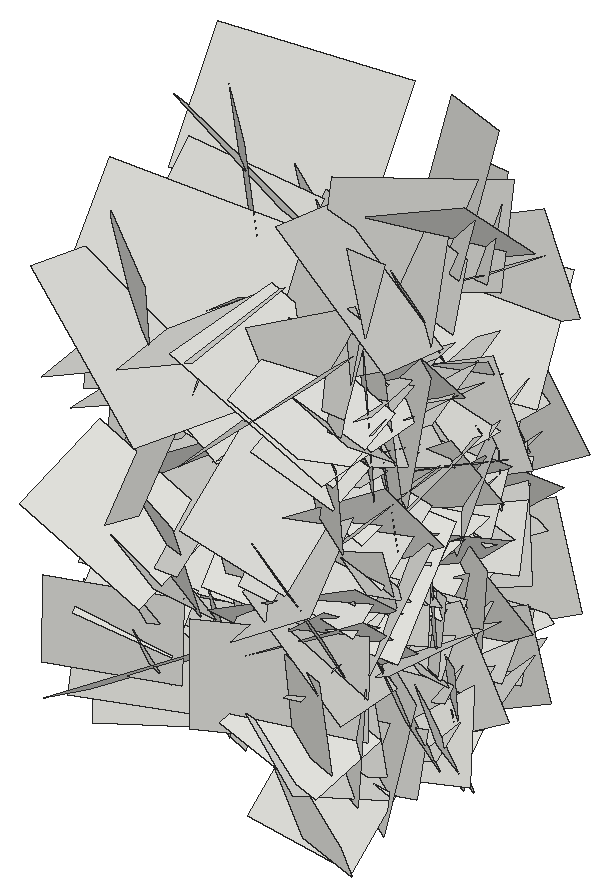
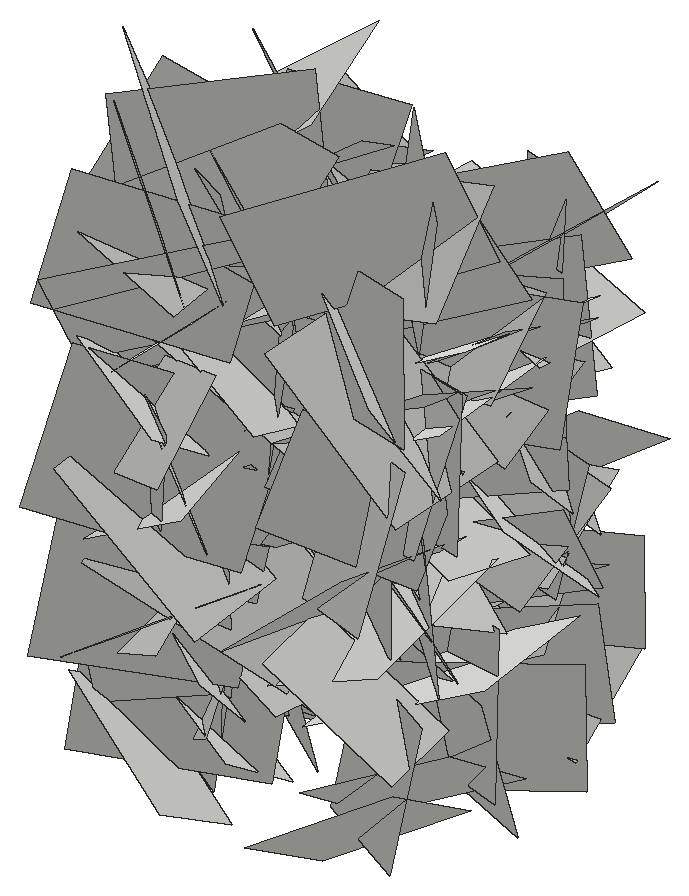
# SketchUp Ruby script. Lengths in inches.
U = 1.inch
M = Sketchup.active_model
def pt(a) = Geom::Point3d.new(a.map { |v| v * U })
def face(e, loops, mat)
  f = e.add_face(loops[0].map { |a| pt(a) })
  loops[1..].each { |l| e.add_face(l.map { |a| pt(a) }).erase! }
  f.material = f.back_material = mat if mat
  f
end
# faces: each face lists its corners as indices into pts; further lists are holes
def faces(e, pts, list, mat = nil) = list.each { |f| face(e, (f[0].is_a?(Array) ? f : [f]).map { |l| l.map { |i| pts[i] } }, mat) }
# xy, xz, yz: faces in a plane at the given z, y or x. An outline is a flat list of corners, or four numbers for a rectangle; further outlines are holes
def ring(l) = l.size == 4 ? [[l[0], l[1]], [l[2], l[1]], [l[2], l[3]], [l[0], l[3]]] : l.each_slice(2).to_a
def flat(e, list, mat, &to3) = list.each { |f| face(e, (f[0].is_a?(Array) ? f : [f]).map { |l| ring(l).map { |u, v| to3.(u, v) } }, mat) }
def xy(e, z, list, mat = nil) = flat(e, list, mat) { |x, y| [x, y, z] }
def xz(e, y, list, mat = nil) = flat(e, list, mat) { |x, z| [x, y, z] }
def yz(e, x, list, mat = nil) = flat(e, list, mat) { |y, z| [x, y, z] }
def lines(e, pts, list) = list.each { |a, b| e.add_line(pt(pts[a]), pt(pts[b])) }
# prism: a flat outline (further loops are holes) pulled along v
def prism(e, loops, v, mat = nil)
  f = face(e, loops, mat); d = Geom::Vector3d.new(v.map { |x| x * U })
  f.pushpull(f.normal.samedirection?(d) ? d.length : -d.length)
end
def box(e, o, s, mat = nil) = prism(e, [[o, [o[0] + s[0], o[1], o[2]], [o[0] + s[0], o[1] + s[1], o[2]], [o[0], o[1] + s[1], o[2]]]], [0, 0, s[2]], mat)
def at(x, y, z, deg = 0) = Geom::Transformation.translation(pt([x, y, z])) * Geom::Transformation.rotation(ORIGIN, Z_AXIS, deg.degrees)
def axes(o, x, y, z) = Geom::Transformation.new([*x, 0, *y, 0, *z, 0, *pt(o).to_a, 1])
def part(name) = M.definitions.add(name)
# library, detail: a bought-in or finely detailed component or shape, given as its bounding box
def library(name, o, s) = part(name).tap { |d| box(d.entities, o, s) }
def detail(e, o, s) = box(e.add_group.entities, o, s)
def put(e, d, t, mat = nil) = e.add_instance(d, t).tap { |i| i.material = mat if mat }
def group(e, t, mat = nil) = e.add_group.tap { |g| g.transformation = t; g.material = mat if mat }.entities
root = M.entities
c1 = part("Component\#6")
p = [[0.01,0,0],[0,3.24,4.54],[4.32,3.24,4.54],[4.33,0,0]]
faces(c1.entities,p,[[0,1,2,3]])
put(root,c1,axes([404.88,151.13,9.12],[0.15296,0.67587,0.31221],[-0.03502,0.32352,-0.68509],[-0.78839,0.11676,0.09101]))
put(root,c1,axes([400.91,158.45,22.43],[-0.19892,0.24365,-1.12098],[0.08242,-1.13056,-0.25875],[1.21318,0.11676,-0.16622]))
put(root,c1,axes([400.91,153.47,7.93],[-0.25077,0.36385,-1.26635],[-0.08689,-1.28818,-0.35481],[1.39394,-0.01484,-0.24993]))
put(root,c1,axes([404.88,151.91,13.09],[0.06029,-0.61389,0.14039],[-0.0496,0.13645,0.61563],[-0.66568,-0.06576,-0.03315]))
put(root,c1,axes([404.88,155.37,8.05],[0.03179,-0.04018,0.69029],[0.07893,0.6871,0.03676],[-0.72868,0.07267,0.03409]))
put(root,c1,axes([404.88,147.25,18.09],[0.11506,-0.20062,0.68841],[0.02156,0.69683,0.19986],[-0.75976,-0.01061,0.10993]))
put(root,c1,axes([404.88,146,16.15],[0.10062,0.63244,0.10884],[-0.07256,0.11937,-0.63396],[-0.67636,0.08128,0.0842]))
put(root,c1,axes([400.91,157.74,11.21],[0.0595,-0.6331,0.72554],[0.06262,0.72766,0.63038],[1.01877,-0.00775,-0.08112]))
put(root,c1,axes([400.91,160.22,19.0625],[-0.13961,-0.68099,-1.03193],[-0.07146,-1.03227,0.68982],[1.30861,-0.12902,-0.07242]))
put(root,c1,axes([404.88,149.02,5.32],[0.19432,-0.67994,0.40742],[0.04988,0.42677,0.69106],[-0.83874,-0.13215,0.13549]))
put(root,c1,axes([400.91,154.9,1.8],[0.03269,0.90387,0.50014],[0.00572,0.50021,-0.90434],[1.09498,-0.0296,-0.01021]))
put(root,c1,axes([404.88,152.72,13.34],[0.14332,-0.62648,-0.12325],[-0.10799,-0.14554,0.62801],[-0.66813,-0.11086,-0.12794]))
put(root,c1,axes([400.91,157.43,12.97],[-0.1074,-0.05602,-1.35571],[-0.22854,-1.34155,0.07155],[1.42001,-0.22014,-0.09102]))
put(root,c1,axes([400.91,151.01,19.39],[0.01021,0.65154,-0.69294],[0.23408,-0.67557,-0.63214],[0.98066,0.15447,0.1581]))
put(root,c1,axes([400.91,148.31,17.26],[0.09379,0.98835,0.28145],[-0.01751,0.28383,-0.99149],[1.08916,-0.08054,-0.04018]))
put(root,c1,axes([400.91,155.4,17.52],[-0.19723,0.3027,-1.19403],[0.0763,-1.20284,-0.31615],[1.30348,0.11621,-0.16216]))
put(root,c1,axes([400.91,145.87,3.84],[0.08046,-0.07863,0.91675],[0.19442,0.90269,0.06223],[0.95574,-0.17701,-0.08983]))
put(root,c1,axes([400.91,148.09,7.11],[-0.15706,0.67864,1.02073],[0.03183,1.02986,-0.68036],[1.29889,0.05683,0.1401]))
put(root,c1,axes([400.91,148.93,-0.125],[-0.17085,0.2332,1.25619],[-0.02467,1.2654,-0.2379],[1.35409,0.05247,0.15416]))
put(root,c1,axes([400.91,158.83,13.98],[0.00743,-1.2386,0.03478],[-0.17851,0.0335,1.22715],[1.30124,0.01167,0.16814]))
put(root,c1,axes([400.91,152.08,1.74],[0.04493,0.85391,0.54577],[0.09586,0.54089,-0.85328],[1.06994,-0.08432,0.05353]))
put(root,c1,axes([400.91,151.75,19.45],[0.16935,0.44212,0.83371],[0.05466,0.84022,-0.45546],[0.99881,-0.12095,-0.11643]))
put(root,c1,axes([404.88,150.18,6.375],[0.17639,-0.58204,-0.33942],[-0.00316,-0.35025,0.59915],[-0.71419,-0.1422,-0.08648]))
put(root,c1,axes([404.88,148.65,3.04],[0.12439,-0.47488,0.46679],[0.05284,0.47892,0.47469],[-0.70386,-0.04797,0.11813]))
put(root,c1,axes([400.91,156.6875,24.44],[0.16473,0.01802,-1.18121],[-0.23771,-1.16927,-0.04735],[1.22945,-0.22849,0.14911]))
put(root,c1,axes([400.91,147.43,1.76],[0.0449,0.15818,1.07958],[0.0304,1.07985,-0.15935],[1.15617,-0.03454,-0.03773]))
put(root,c1,axes([400.91,158.38,15.93],[-0.03304,0.59909,-1.16183],[-0.1621,-1.15585,-0.5919],[1.37611,-0.12177,-0.09762]))
put(root,c1,axes([400.91,156.09,10.89],[0.02844,-1.01096,-0.23497],[0.17327,-0.228,0.99963],[1.08645,0.06282,-0.15327]))
put(root,c1,axes([400.91,159.05,4.5],[0.22831,-0.97739,-0.02602],[-0.01319,-0.02938,1.00067],[1.03632,0.21495,0.01847]))
put(root,c1,axes([400.91,157.5,5.99],[0.02733,0.34478,-1.12821],[-0.04378,-1.12752,-0.34552],[1.24973,-0.04704,0.01257]))
put(root,c1,axes([400.91,147.25,11.15],[0.01251,0.83252,-0.66438],[0.16644,-0.65852,-0.82239],[1.1167,0.08883,0.13002]))
put(root,c1,axes([400.91,153.16,13.74],[0.07693,-1.07175,0.44962],[-0.07215,0.4458,1.07364],[1.22986,0.09319,0.03486]))
put(root,c1,axes([400.91,150.33,13.2],[-0.24126,0.02501,1.36725],[0.05252,1.3853,-0.01709],[1.44858,-0.04606,0.22834]))
put(root,c1,axes([400.91,144.59,11.1],[0.20686,0.83944,0.54314],[0.00436,0.55271,-0.85571],[1.05982,-0.16612,-0.10249]))
put(root,c1,axes([400.91,153.72,24.55],[-0.10736,0.8301,-0.78481],[0.26067,-0.75358,-0.8288],[1.18252,0.24148,0.11144]))
put(root,c1,axes([400.91,148.8125,12.02],[0.02959,0.36254,-1.01381],[0.21176,-0.99828,-0.35148],[1.12146,0.17893,0.09312]))
put(root,c1,axes([400.91,148.37,14.37],[0.13394,0.02599,1.3483],[-0.3112,1.32226,0.00203],[1.39518,0.29244,-0.12899]))
put(root,c1,axes([400.91,151.84,12.71],[0.09641,-0.969,-0.91768],[-0.24854,-0.9171,0.94515],[1.39265,-0.09659,0.2322]))
put(root,c1,axes([400.91,152.41,8.09],[-0.02535,-1.06677,0.60381],[0.0625,0.60222,1.06631],[1.29785,-0.04984,-0.03955]))
put(root,c1,axes([400.91,153.41,21.56],[0.04666,0.60871,1.19242],[-0.17987,1.18598,-0.59916],[1.40769,0.13136,-0.11609]))
put(root,c1,axes([400.91,154.4,5.48],[-0.14525,-0.2612,-1.20099],[0.27145,-1.18798,0.22915],[1.27422,0.2233,-0.18571]))
put(root,c1,axes([400.91,153.21,11.43],[-0.14123,-0.96535,-0.93141],[0.15435,-0.94087,0.95433],[1.41351,0.00629,-0.19727]))
put(root,c1,axes([400.91,157.09,9.16],[0.26081,-0.66319,-0.77037],[0.09697,-0.77495,0.69635],[1.07312,0.23121,0.12431]))
put(root,c1,axes([400.91,149.27,6.59],[-0.15688,1.33929,-0.00269],[0.18956,0.01708,-1.33541],[1.40693,0.14704,0.17962]))
put(root,c1,axes([400.91,149.82,11.51],[0.16938,-0.10345,1.35904],[-0.25816,1.34416,0.13095],[1.4215,0.25644,-0.13816]))
put(root,c1,axes([400.91,155.16,12.125],[0.20792,1.23942,0.0793],[-0.14973,0.10203,-1.24521],[1.30793,-0.18535,-0.15516]))
put(root,c1,axes([400.91,151.77,16.16],[0.14743,1.12249,0.38129],[0.0578,0.37744,-1.13105],[1.25528,-0.14922,0.00729]))
put(root,c1,axes([400.91,145.22,20.96],[0.20751,1.35949,-0.09859],[-0.20583,-0.07077,-1.36145],[1.43011,-0.20745,-0.18164]))
put(root,c1,axes([400.91,149.47,1.18],[0.22795,-1.08393,0.44752],[0.03192,0.45993,1.09954],[1.24263,0.18702,-0.11034]))
put(root,c1,axes([400.91,155.15,17.37],[0.02517,0.60882,-1.16754],[0.2041,-1.15679,-0.59929],[1.38075,0.1599,0.10987]))
put(root,c1,axes([400.91,146.56,18.67],[0.08115,0.67304,1.19325],[0.03541,1.19384,-0.67552],[1.45175,-0.06674,-0.05023]))
put(root,c1,axes([400.91,150.46,17.01],[0.04698,1.34267,-0.16756],[0.13374,-0.17102,-1.33703],[1.42802,-0.02815,0.13073]))
put(root,c1,axes([400.91,150.02,13.53],[0.11354,-0.10924,1.28227],[0.18202,1.27641,0.09439],[1.35193,-0.16268,-0.1204]))
put(root,c1,axes([400.91,153.54,10.59],[0.17173,1.22834,-0.55665],[0.01226,-0.5619,-1.23655],[1.42944,-0.14275,0.07748]))
put(root,c1,axes([400.91,151.36,16.73],[0.05564,-1.33407,-0.12972],[0.26745,-0.11766,1.31218],[1.39538,0.07575,-0.24633]))
put(root,c1,axes([400.91,148.21,18.05],[0.18781,1.38239,0.05917],[0.11095,0.04609,-1.39025],[1.46247,-0.18102,0.09787]))
put(root,c1,axes([414.68,148.21,18.05],[-0.18781,1.38239,0.05917],[-0.11095,0.04609,-1.39025],[-1.46247,-0.18102,0.09787]))
put(root,c1,axes([414.68,151.36,16.73],[-0.05564,-1.33407,-0.12972],[-0.26745,-0.11766,1.31218],[-1.39538,0.07575,-0.24633]))
put(root,c1,axes([414.68,153.54,10.59],[-0.17173,1.22834,-0.55665],[-0.01226,-0.5619,-1.23655],[-1.42944,-0.14275,0.07748]))
put(root,c1,axes([414.68,150.02,13.53],[-0.11354,-0.10924,1.28227],[-0.18202,1.27641,0.09439],[-1.35193,-0.16268,-0.1204]))
put(root,c1,axes([414.68,150.46,17.01],[-0.04698,1.34267,-0.16756],[-0.13374,-0.17102,-1.33703],[-1.42802,-0.02815,0.13073]))
put(root,c1,axes([414.68,146.56,18.67],[-0.08115,0.67304,1.19325],[-0.03541,1.19384,-0.67552],[-1.45175,-0.06674,-0.05023]))
put(root,c1,axes([414.68,155.15,17.37],[-0.02517,0.60882,-1.16754],[-0.2041,-1.15679,-0.59929],[-1.38075,0.1599,0.10987]))
put(root,c1,axes([414.68,149.47,1.18],[-0.22795,-1.08393,0.44752],[-0.03192,0.45993,1.09954],[-1.24263,0.18702,-0.11034]))
put(root,c1,axes([414.68,145.22,20.96],[-0.20751,1.35949,-0.09859],[0.20583,-0.07077,-1.36145],[-1.43011,-0.20745,-0.18164]))
put(root,c1,axes([414.68,151.77,16.16],[-0.14743,1.12249,0.38129],[-0.0578,0.37744,-1.13105],[-1.25528,-0.14922,0.00729]))
put(root,c1,axes([414.68,155.16,12.125],[-0.20792,1.23942,0.0793],[0.14973,0.10203,-1.24521],[-1.30793,-0.18535,-0.15516]))
put(root,c1,axes([414.68,149.82,11.51],[-0.16938,-0.10345,1.35904],[0.25816,1.34416,0.13095],[-1.4215,0.25644,-0.13816]))
put(root,c1,axes([414.68,149.27,6.59],[0.15688,1.33929,-0.00269],[-0.18956,0.01708,-1.33541],[-1.40693,0.14704,0.17962]))
put(root,c1,axes([414.68,157.09,9.16],[-0.26081,-0.66319,-0.77037],[-0.09697,-0.77495,0.69635],[-1.07312,0.23121,0.12431]))
put(root,c1,axes([414.68,153.21,11.43],[0.14123,-0.96535,-0.93141],[-0.15435,-0.94087,0.95433],[-1.41351,0.00629,-0.19727]))
put(root,c1,axes([414.68,148.05,8.79],[-0.07068,0.0827,-1.14811],[-0.1221,-1.14474,-0.07576],[-1.21402,0.11031,0.07447]))
put(root,c1,axes([414.68,154.4,5.48],[0.14525,-0.2612,-1.20099],[-0.27145,-1.18798,0.22915],[-1.27422,0.2233,-0.18571]))
put(root,c1,axes([414.68,153.41,21.56],[-0.04666,0.60871,1.19242],[0.17987,1.18598,-0.59916],[-1.40769,0.13136,-0.11609]))
put(root,c1,axes([414.68,152.41,8.09],[0.02535,-1.06677,0.60381],[-0.0625,0.60222,1.06631],[-1.29785,-0.04984,-0.03955]))
put(root,c1,axes([414.68,151.84,12.71],[-0.09641,-0.969,-0.91768],[0.24854,-0.9171,0.94515],[-1.39265,-0.09659,0.2322]))
put(root,c1,axes([414.68,148.37,14.37],[-0.13394,0.02599,1.3483],[0.3112,1.32226,0.00203],[-1.39518,0.29244,-0.12899]))
put(root,c1,axes([414.68,148.8125,12.02],[-0.02959,0.36254,-1.01381],[-0.21176,-0.99828,-0.35148],[-1.12146,0.17893,0.09312]))
put(root,c1,axes([414.68,153.72,24.55],[0.10736,0.8301,-0.78481],[-0.26067,-0.75358,-0.8288],[-1.18252,0.24148,0.11144]))
put(root,c1,axes([414.68,144.59,11.1],[-0.20686,0.83944,0.54314],[-0.00436,0.55271,-0.85571],[-1.05982,-0.16612,-0.10249]))
put(root,c1,axes([414.68,150.33,13.2],[0.24126,0.02501,1.36725],[-0.05252,1.3853,-0.01709],[-1.44858,-0.04606,0.22834]))
put(root,c1,axes([414.68,153.16,13.74],[-0.07693,-1.07175,0.44962],[0.07215,0.4458,1.07364],[-1.22986,0.09319,0.03486]))
put(root,c1,axes([414.68,147.25,11.15],[-0.01251,0.83252,-0.66438],[-0.16644,-0.65852,-0.82239],[-1.1167,0.08883,0.13002]))
put(root,c1,axes([414.68,157.5,5.99],[-0.02733,0.34478,-1.12821],[0.04378,-1.12752,-0.34552],[-1.24973,-0.04704,0.01257]))
put(root,c1,axes([414.68,159.05,4.5],[-0.22831,-0.97739,-0.02602],[0.01319,-0.02938,1.00067],[-1.03632,0.21495,0.01847]))
put(root,c1,axes([414.68,156.09,10.89],[-0.02844,-1.01096,-0.23497],[-0.17327,-0.228,0.99963],[-1.08645,0.06282,-0.15327]))
put(root,c1,axes([414.68,158.38,15.93],[0.03304,0.59909,-1.16183],[0.1621,-1.15585,-0.5919],[-1.37611,-0.12177,-0.09762]))
put(root,c1,axes([414.68,147.43,1.76],[-0.0449,0.15818,1.07958],[-0.0304,1.07985,-0.15935],[-1.15617,-0.03454,-0.03773]))
put(root,c1,axes([414.68,156.6875,24.44],[-0.16473,0.01802,-1.18121],[0.23771,-1.16927,-0.04735],[-1.22945,-0.22849,0.14911]))
put(root,c1,axes([410.71,148.65,3.04],[-0.12439,-0.47488,0.46679],[-0.05284,0.47892,0.47469],[0.70386,-0.04797,0.11813]))
put(root,c1,axes([410.71,150.18,6.375],[-0.17639,-0.58204,-0.33942],[0.00316,-0.35025,0.59915],[0.71419,-0.1422,-0.08648]))
put(root,c1,axes([414.68,151.75,19.45],[-0.16935,0.44212,0.83371],[-0.05466,0.84022,-0.45546],[-0.99881,-0.12095,-0.11643]))
put(root,c1,axes([414.68,152.08,1.74],[-0.04493,0.85391,0.54577],[-0.09586,0.54089,-0.85328],[-1.06994,-0.08432,0.05353]))
put(root,c1,axes([414.68,158.83,13.98],[-0.00743,-1.2386,0.03478],[0.17851,0.0335,1.22715],[-1.30124,0.01167,0.16814]))
put(root,c1,axes([414.68,148.93,-0.125],[0.17085,0.2332,1.25619],[0.02467,1.2654,-0.2379],[-1.35409,0.05247,0.15416]))
put(root,c1,axes([414.68,148.09,7.11],[0.15706,0.67864,1.02073],[-0.03183,1.02986,-0.68036],[-1.29889,0.05683,0.1401]))
put(root,c1,axes([414.68,145.87,3.84],[-0.08046,-0.07863,0.91675],[-0.19442,0.90269,0.06223],[-0.95574,-0.17701,-0.08983]))
put(root,c1,axes([414.68,155.4,17.52],[0.19723,0.3027,-1.19403],[-0.0763,-1.20284,-0.31615],[-1.30348,0.11621,-0.16216]))
put(root,c1,axes([414.68,148.31,17.26],[-0.09379,0.98835,0.28145],[0.01751,0.28383,-0.99149],[-1.08916,-0.08054,-0.04018]))
put(root,c1,axes([414.68,151.01,19.39],[-0.01021,0.65154,-0.69294],[-0.23408,-0.67557,-0.63214],[-0.98066,0.15447,0.1581]))
put(root,c1,axes([414.68,157.43,12.97],[0.1074,-0.05602,-1.35571],[0.22854,-1.34155,0.07155],[-1.42001,-0.22014,-0.09102]))
put(root,c1,axes([410.71,152.72,13.34],[-0.14332,-0.62648,-0.12325],[0.10799,-0.14554,0.62801],[0.66813,-0.11086,-0.12794]))
put(root,c1,axes([414.68,154.9,1.8],[-0.03269,0.90387,0.50014],[-0.00572,0.50021,-0.90434],[-1.09498,-0.0296,-0.01021]))
put(root,c1,axes([410.71,149.02,5.32],[-0.19432,-0.67994,0.40742],[-0.04988,0.42677,0.69106],[0.83874,-0.13215,0.13549]))
put(root,c1,axes([414.68,160.22,19.0625],[0.13961,-0.68099,-1.03193],[0.07146,-1.03227,0.68982],[-1.30861,-0.12902,-0.07242]))
put(root,c1,axes([414.68,157.74,11.21],[-0.0595,-0.6331,0.72554],[-0.06262,0.72766,0.63038],[-1.01877,-0.00775,-0.08112]))
put(root,c1,axes([410.71,146,16.15],[-0.10062,0.63244,0.10884],[0.07256,0.11937,-0.63396],[0.67636,0.08128,0.0842]))
put(root,c1,axes([410.71,147.25,18.09],[-0.11506,-0.20062,0.68841],[-0.02156,0.69683,0.19986],[0.75976,-0.01061,0.10993]))
put(root,c1,axes([410.71,155.37,8.05],[-0.03179,-0.04018,0.69029],[-0.07893,0.6871,0.03676],[0.72868,0.07267,0.03409]))
put(root,c1,axes([410.71,151.91,13.09],[-0.06029,-0.61389,0.14039],[0.0496,0.13645,0.61563],[0.66568,-0.06576,-0.03315]))
put(root,c1,axes([414.68,153.47,7.93],[0.25077,0.36385,-1.26635],[0.08689,-1.28818,-0.35481],[-1.39394,-0.01484,-0.24993]))
put(root,c1,axes([414.68,158.45,22.43],[0.19892,0.24365,-1.12098],[-0.08242,-1.13056,-0.25875],[-1.21318,0.11676,-0.16622]))
put(root,c1,axes([410.71,151.13,9.12],[-0.15296,0.67587,0.31221],[0.03502,0.32352,-0.68509],[0.78839,0.11676,0.09101]))
put(root,c1,axes([414.68,148.76,4.0625],[-0.10183,-0.75916,-0.2873],[-0.20096,-0.26032,0.75126],[-0.83661,0.15493,-0.14549]))
put(root,c1,axes([414.68,155.05,20.66],[-0.11898,0.43702,0.87755],[0.10329,0.88388,-0.42771],[-1.03402,0.038,-0.1437]))
put(root,c1,axes([414.68,154.79,8.7],[0.06507,0.61236,-0.89404],[0.03144,-0.89608,-0.61173],[-1.14823,0.01016,-0.06741]))
put(root,c1,axes([410.71,151.99,2.12],[-0.1775,0.68354,0.35821],[0.06031,0.37649,-0.69181],[0.81579,0.12089,0.12909]))
put(root,c1,axes([410.71,151.79,4.27],[-0.00282,-0.67031,0.14172],[-0.04158,0.14164,0.66918],[0.72504,0.00552,0.03892]))
put(root,c1,axes([410.71,147.62,1.41],[-0.08717,-0.06025,0.7019],[0.04865,0.70471,0.06586],[0.74517,-0.05306,0.07781]))
put(root,c1,axes([410.71,156.87,7.65],[0.00449,0.50233,-0.39291],[0.02578,-0.39276,-0.50188],[0.67552,0.01165,0.02176]))
put(root,c1,axes([410.71,153.92,20.8125],[0.01755,0.277,-0.54123],[0.05617,-0.54003,-0.27476],[0.64202,0.03967,0.03883]))
put(root,c1,axes([414.68,152.6,3.91],[-0.02426,0.68313,0.69515],[0.0107,0.69547,-0.68312],[-1.03305,-0.00884,-0.0234]))
put(root,c1,axes([410.71,147.13,6.96],[-0.04816,-0.19283,0.63159],[0.07038,0.62854,0.19668],[0.69645,-0.07685,0.0238]))
put(root,c1,axes([414.68,158.68,8.63],[0.07829,-0.94373,0.27717],[-0.10215,0.26967,0.94388],[-1.03759,-0.09775,-0.07202]))
put(root,c1,axes([414.68,152.91,14.99],[0.05042,0.65822,-0.8803],[0.11398,-0.87969,-0.65195],[-1.15954,-0.05785,-0.10236]))
put(root,c1,axes([414.68,159.16,9.85],[0.13765,0.1916,-1.18129],[0.14512,-1.1828,-0.17679],[-1.2602,-0.11528,-0.14939]))
put(root,c1,axes([414.68,157.06,14.03],[0.04606,-0.47436,-0.98882],[0.12961,-0.98133,0.47614],[-1.15527,-0.12901,0.01399]))
put(root,c1,axes([414.68,149.64,15.49],[0.05397,-0.71515,0.49033],[-0.26351,0.45852,0.69456],[-0.88054,-0.18105,-0.1778]))
put(root,c1,axes([410.71,148.39,13.69],[0.056,0.56116,0.2115],[0.06403,0.20626,-0.56234],[0.63244,-0.07057,0.03821]))
put(root,c1,axes([414.68,147.71,9.53],[0.0202,0.73421,-0.62443],[-0.01239,-0.62433,-0.73445],[-1.02159,0.02209,-0.00344]))
put(root,c1,axes([410.71,146.72,8.375],[0.05548,0.31048,0.67068],[-0.12303,0.66747,-0.29994],[0.77368,0.08387,-0.09579]))
put(root,c1,axes([414.68,152.28,1.18],[0.22482,-0.75958,0.923],[0.06114,0.94282,0.76264],[-1.2656,-0.08938,0.2008]))
put(root,c1,axes([414.68,154.73,4.99],[0.23466,-0.21907,1.02966],[-0.17179,1.03255,0.25453],[-1.10257,-0.20751,0.17949]))
put(root,c1,axes([410.71,148.44,10.1],[0.02371,0.59128,0.15103],[0.13632,0.14317,-0.57956],[0.63236,-0.05303,0.11928]))
put(root,c1,axes([410.71,154.81,5.31],[0.03271,-0.68931,-0.29186],[-0.0897,-0.29345,0.68411],[0.78838,-0.00479,0.08995]))
put(root,c1,axes([410.71,155.07,5.6],[-0.26442,-0.95782,0.42161],[-0.12666,0.45666,0.96674],[1.10204,-0.17733,0.21227]))
put(root,c1,axes([414.68,146.38,17.95],[-0.09245,0.38694,0.78979],[0.04684,0.79459,-0.38441],[-0.93107,0.00155,-0.09776]))
put(root,c1,axes([410.71,155.43,2.74],[0.05213,0.12024,0.7107],[-0.06472,0.71048,-0.11598],[0.7613,0.05216,-0.05853]))
put(root,c1,axes([414.68,149.03,14.67],[0.12882,0.64149,-0.81464],[-0.00451,-0.8199,-0.64626],[-1.09909,0.07855,-0.09282]))
put(root,c1,axes([410.71,145.53,10.42],[-0.22479,1.04725,-0.16356],[-0.16331,-0.19548,-1.05191],[1.11161,0.18306,-0.18761]))
put(root,c1,axes([414.68,147.21,13.43],[0.06341,1.09172,0.23851],[0.19798,0.22572,-1.08003],[-1.16785,0.09755,-0.17015]))
put(root,c1,axes([410.71,146.09,12.1875],[-0.18427,0.52878,-0.65011],[0.11203,-0.64482,-0.55274],[0.8812,0.19255,-0.06567]))
put(root,c1,axes([414.68,151.57,3.27],[-0.14157,0.02397,-0.74069],[-0.04702,-0.75154,-0.01632],[-0.78414,0.04073,0.1347]))
put(root,c1,axes([410.71,154.48,3.89],[0.11783,0.23417,0.69133],[-0.11259,0.69704,-0.21902],[0.76547,0.06648,-0.13863]))
put(root,c1,axes([410.71,152.53,7.1875],[0.08757,-0.64703,0.3684],[-0.09594,0.35919,0.65114],[0.78338,0.11632,0.03856]))
put(root,c1,axes([414.68,153.68,-0.24],[-0.08313,-0.05331,0.78078],[-0.05564,0.78328,0.04821],[-0.82769,-0.0473,-0.08166]))
put(root,c1,axes([410.71,155.23,10.47],[-0.04155,0.12694,-0.87349],[-0.11983,-0.86787,-0.12105],[0.92792,-0.10639,-0.05475]))
put(root,c1,axes([414.68,154.93,13.48],[0.13332,0.92748,-0.67904],[0.1887,-0.69057,-0.91025],[-1.20375,-0.00553,-0.2179]))
put(root,c1,axes([414.68,152.46,19.1],[0.24316,-1.11668,0.32256],[0.08367,0.34299,1.13127],[-1.22923,-0.19755,0.14081]))
put(root,c1,axes([414.68,149.625,17.57],[-0.05592,-0.7816,-0.40589],[0.0657,-0.4089,0.77935],[-0.93124,0.01809,0.07936]))
put(root,c1,axes([410.71,153.02,6.56],[0.04835,0.51462,-0.41299],[0.10228,-0.41473,-0.50612],[0.69191,0.02534,0.10368]))
put(root,c1,axes([410.71,155.74,21.65],[-0.00825,-0.17983,-0.66547],[0.14401,-0.65286,0.17483],[0.71636,0.12918,-0.04281]))
put(root,c1,axes([414.68,147.06,-0.97],[-0.01135,-0.66277,0.66685],[0.09721,0.66298,0.66039],[-0.99185,0.07256,0.05709]))
put(root,c1,axes([410.71,154.86,6.54],[-0.11481,0.21277,-0.79232],[0.09254,-0.79167,-0.22453],[0.86468,0.11298,-0.08117]))
put(root,c1,axes([414.68,155.95,10.68],[-0.04823,-0.00518,0.84226],[0.02844,0.84305,0.00663],[-0.89236,0.02715,-0.04531]))
put(root,c1,axes([414.68,146.53,12.92],[-0.03124,-0.05121,0.8385],[0.00373,0.839,0.05136],[-0.89046,0.00531,-0.0292]))
put(root,c1,axes([414.68,152.8,10.75],[0.04843,-0.82009,-0.82841],[0.32646,-0.79109,0.80013],[-1.19171,-0.25004,0.18553]))
put(root,c1,axes([410.71,155.82,10.86],[-0.10869,-0.77244,0.23734],[0.13092,0.22145,0.77409],[0.8465,-0.13343,-0.08925]))
put(root,c1,axes([410.71,156.49,11.61],[-0.16435,-0.92659,-0.48849],[-0.14398,-0.47186,0.93815],[1.10094,-0.20004,0.04977]))
put(root,c1,axes([414.68,153.88,7.81],[-0.12498,-0.19712,-0.75186],[0.05107,-0.76085,0.19192],[-0.82232,-0.01729,0.12619]))
put(root,c1,axes([410.71,154.72,7.86],[0.01434,-0.12328,-0.7123],[0.10241,-0.70572,0.12398],[0.75939,0.0975,-0.00327]))
put(root,c1,axes([414.68,155.22,14.18],[0.0107,0.67836,0.43703],[-0.08223,0.43585,-0.67474],[-0.8514,-0.03357,0.07066]))
put(root,c1,axes([410.71,152.55,8.85],[-0.17208,0.39932,0.93109],[-0.08126,0.93542,-0.41455],[1.07081,0.13515,0.11817]))
put(root,c1,axes([414.68,155.14,21.07],[0.01676,0.7943,-0.14622],[-0.08914,-0.14383,-0.79043],[-0.85145,0.03069,0.07988]))
put(root,c1,axes([410.71,158.76,13.54],[-0.17018,-0.33172,-0.9968],[-0.1229,-0.99662,0.35033],[1.10678,-0.16167,-0.11436]))
put(root,c1,axes([414.68,151.77,10.3],[-0.00621,-0.04081,-0.81439],[-0.02737,-0.814,0.04098],[-0.86391,0.02608,0.00455]))
put(root,c1,axes([414.68,149.67,1.32],[-0.10197,-0.47157,-0.58691],[0.00963,-0.59236,0.47447],[-0.798,0.05311,0.08072]))
put(root,c1,axes([410.71,154.27,5.56],[-0.10843,0.64197,-0.78685],[-0.13439,-0.79271,-0.63027],[1.06801,-0.03458,-0.15919]))
